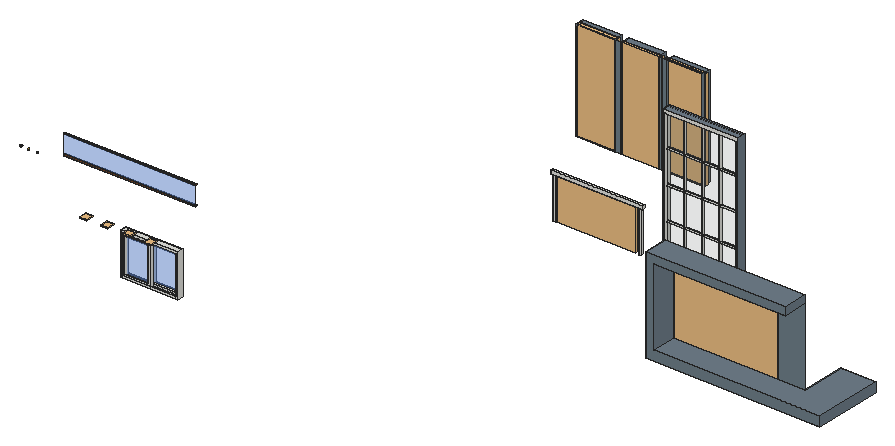
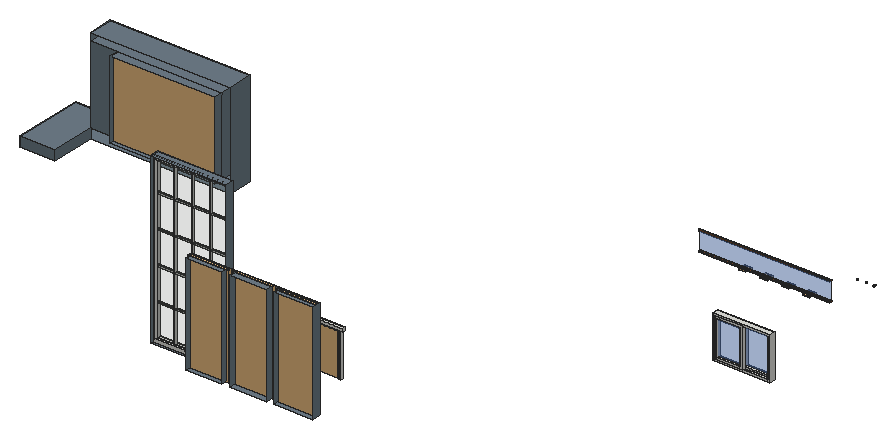
# SketchUp Ruby script. Lengths in inches.
U = 1.inch
M = Sketchup.active_model
def pt(a) = Geom::Point3d.new(a.map { |v| v * U })
def face(e, loops, mat)
  f = e.add_face(loops[0].map { |a| pt(a) })
  loops[1..].each { |l| e.add_face(l.map { |a| pt(a) }).erase! }
  f.material = f.back_material = mat if mat
  f
end
# faces: each face lists its corners as indices into pts; further lists are holes
def faces(e, pts, list, mat = nil) = list.each { |f| face(e, (f[0].is_a?(Array) ? f : [f]).map { |l| l.map { |i| pts[i] } }, mat) }
# xy, xz, yz: faces in a plane at the given z, y or x. An outline is a flat list of corners, or four numbers for a rectangle; further outlines are holes
def ring(l) = l.size == 4 ? [[l[0], l[1]], [l[2], l[1]], [l[2], l[3]], [l[0], l[3]]] : l.each_slice(2).to_a
def flat(e, list, mat, &to3) = list.each { |f| face(e, (f[0].is_a?(Array) ? f : [f]).map { |l| ring(l).map { |u, v| to3.(u, v) } }, mat) }
def xy(e, z, list, mat = nil) = flat(e, list, mat) { |x, y| [x, y, z] }
def xz(e, y, list, mat = nil) = flat(e, list, mat) { |x, z| [x, y, z] }
def yz(e, x, list, mat = nil) = flat(e, list, mat) { |y, z| [x, y, z] }
def lines(e, pts, list) = list.each { |a, b| e.add_line(pt(pts[a]), pt(pts[b])) }
# prism: a flat outline (further loops are holes) pulled along v
def prism(e, loops, v, mat = nil)
  f = face(e, loops, mat); d = Geom::Vector3d.new(v.map { |x| x * U })
  f.pushpull(f.normal.samedirection?(d) ? d.length : -d.length)
end
def box(e, o, s, mat = nil) = prism(e, [[o, [o[0] + s[0], o[1], o[2]], [o[0] + s[0], o[1] + s[1], o[2]], [o[0], o[1] + s[1], o[2]]]], [0, 0, s[2]], mat)
def at(x, y, z, deg = 0) = Geom::Transformation.translation(pt([x, y, z])) * Geom::Transformation.rotation(ORIGIN, Z_AXIS, deg.degrees)
def axes(o, x, y, z) = Geom::Transformation.new([*x, 0, *y, 0, *z, 0, *pt(o).to_a, 1])
def part(name) = M.definitions.add(name)
# library, detail: a bought-in or finely detailed component or shape, given as its bounding box
def library(name, o, s) = part(name).tap { |d| box(d.entities, o, s) }
def detail(e, o, s) = box(e.add_group.entities, o, s)
def put(e, d, t, mat = nil) = e.add_instance(d, t).tap { |i| i.material = mat if mat }
def group(e, t, mat = nil) = e.add_group.tap { |g| g.transformation = t; g.material = mat if mat }.entities
root = M.entities
M.materials.add("Heather_Cuffs").color = [111, 126, 137]
M.materials.add("[Color D04]").color = [255, 204, 50]
M.materials["[Color D04]"].alpha = 0.66
M.materials.add("[Color E05]").color = [255, 255, 0]
M.materials.add("[Translucent Glass Blue]").color = [100, 149, 237]
M.materials["[Translucent Glass Blue]"].alpha = 0.5
M.materials.add("[Translucent Glass Gray]1").color = [120, 128, 125]
M.materials["[Translucent Glass Gray]1"].alpha = 0.1875
M.materials.add("[Wood Veneer 01]").color = [120, 70, 37]
c1 = part("Group\#58")
box(c1.entities,[0,0,0],[0.79,51.97,0.79])
c2 = part("Group\#67")
box(c2.entities,[0,0,0],[0.79,0.79,79.53])
c3 = part("Group\#8")
xy(c3.entities,0,[[0,0,19.69,39.37]])
c4 = part("Group\#9")
prism(c4.entities,[[[45.28,43.31,0],[45.28,0,0],[21.65,0,0],[21.65,43.31,0]],[[23.62,41.34,0],[23.62,1.97,0],[43.31,1.97,0],[43.31,41.34,0]]],[0,0,1.97])
c5 = part("Group\#13")
g1 = group(c5.entities,at(1.97,1.97,0))
put(g1,c3,at(1.97,1.97,0.98),"[Translucent Glass Blue]")
put(g1,c4,at(-21.65,0,0))
g2 = group(c5.entities,at(23.62,1.97,1.97))
put(g2,c3,at(1.97,1.97,0.98),"[Translucent Glass Blue]")
put(g2,c4,at(-21.65,0,0))
g3 = group(c5.entities,at(0,0,3.9375))
prism(g3,[[[0,47.24,-3.9375],[49.21,47.24,-3.9375],[49.21,0,-3.9375],[0,0,-3.9375]],[[1.97,1.97,-3.9375],[47.24,1.97,-3.9375],[47.24,45.28,-3.9375],[1.97,45.28,-3.9375]]],[0,0,3.9375])
c6 = part("Group43\#1")
box(c6.entities,[916.08,245.78,188.26],[2.36,2.36,22.23])
c7 = part("Group44\#1")
box(c7.entities,[1010.04,245.78,188.26],[2.36,2.36,22.23])
c8 = library("Group47\#1",[920.98,246.17,188.26],[82.61,1.57,22.23])
c9 = library("okno",[0,0,0],[1.97,20.83,48.43])
c10 = library("normal+window",[0,0,0],[4.84,65.35,84.65])
c11 = part("Group46\#1")
box(c11.entities,[916.08,245.58,210.49],[96.32,2.75,1.77])
c12 = part("Group\#7")
box(c12.entities,[0,0,0],[132.53,1.81,1])
prism(root,[[[35.62,61.46,262.86],[35.61,61.72,262.86],[35.68,61.97,262.86],[35.8,62.2,262.86],[35.99,62.39,262.86],[36.21,62.52,262.86],[36.46,62.59,262.86],[36.72,62.6,262.86],[36.97,62.53,262.86],[37.2,62.41,262.86],[37.39,62.22,262.86],[37.52,62,262.86],[37.59,61.75,262.86],[37.6,61.49,262.86],[37.53,61.23,262.86],[37.41,61.01,262.86],[37.23,60.82,262.86],[37,60.68,262.86],[36.75,60.61,262.86],[36.49,60.61,262.86],[36.24,60.67,262.86],[36.01,60.8,262.86],[35.82,60.98,262.86],[35.6875,61.21,262.86]]],[0,0,1],"[Color D04]")
prism(root,[[[26.62,61.46,262.86],[26.61,61.72,262.86],[26.68,61.97,262.86],[26.8,62.2,262.86],[26.99,62.39,262.86],[27.21,62.52,262.86],[27.46,62.59,262.86],[27.72,62.6,262.86],[27.97,62.53,262.86],[28.2,62.41,262.86],[28.39,62.22,262.86],[28.52,62,262.86],[28.59,61.75,262.86],[28.6,61.49,262.86],[28.53,61.23,262.86],[28.41,61.01,262.86],[28.23,60.82,262.86],[28,60.68,262.86],[27.75,60.61,262.86],[27.49,60.61,262.86],[27.24,60.67,262.86],[27.01,60.8,262.86],[26.82,60.98,262.86],[26.6875,61.21,262.86]]],[0,0,1],"[Color D04]")
xy(root,158.93,[[447.88,333.96,522.88,342.96]],"Heather_Cuffs")
xy(root,209.8,[[290.7,420.96,329.6,429.96],[336.74,420.96,373.65,429.96],[381.73,420.96,417.7,429.96]],"Heather_Cuffs")
xy(root,225,[[569.63,194.96,675.0625,203.96]],"Heather_Cuffs")
xy(root,262.86,[[19.49,60.61,19.24,60.67,19.01,60.8,18.82,60.98,18.6875,61.21,18.62,61.46,18.61,61.72,18.68,61.97,18.8,62.2,18.99,62.39,19.21,62.52,19.46,62.59,19.72,62.6,19.97,62.53,20.2,62.41,20.39,62.22,20.52,62,20.59,61.75,20.6,61.49,20.53,61.23,20.41,61.01,20.23,60.82,20,60.68,19.75,60.61]],"[Color D04]")
xy(root,263.86,[[19.49,60.61,19.75,60.61,20,60.68,20.23,60.82,20.41,61.01,20.53,61.23,20.6,61.49,20.59,61.75,20.52,62,20.39,62.22,20.2,62.41,19.97,62.53,19.72,62.6,19.46,62.59,19.21,62.52,18.99,62.39,18.8,62.2,18.68,61.97,18.61,61.72,18.62,61.46,18.6875,61.21,18.82,60.98,19.01,60.8,19.24,60.67]])
xy(root,302,[[586.58,178.82,586.06,178.89,585.58,179.09,585.16,179.41,584.84,179.82,584.64,180.3,584.58,180.82,584.64,181.34,584.84,181.82,585.16,182.23,585.58,182.55,586.06,182.75,586.58,182.82,587.09,182.75,587.58,182.55,587.99,182.23,588.31,181.82,588.51,181.34,588.58,180.82,588.51,180.3,588.31,179.82,587.99,179.41,587.58,179.09,587.09,178.89],[619.58,178.82,619.06,178.89,618.58,179.09,618.16,179.41,617.84,179.82,617.64,180.3,617.58,180.82,617.64,181.34,617.84,181.82,618.16,182.23,618.58,182.55,619.06,182.75,619.58,182.82,620.09,182.75,620.58,182.55,620.99,182.23,621.31,181.82,621.51,181.34,621.58,180.82,621.51,180.3,621.31,179.82,620.99,179.41,620.58,179.09,620.09,178.89],[651.58,178.82,651.06,178.89,650.58,179.09,650.16,179.41,649.84,179.82,649.64,180.3,649.58,180.82,649.64,181.34,649.84,181.82,650.16,182.23,650.58,182.55,651.06,182.75,651.58,182.82,652.09,182.75,652.58,182.55,652.99,182.23,653.31,181.82,653.51,181.34,653.58,180.82,653.51,180.3,653.31,179.82,652.99,179.41,652.58,179.09,652.09,178.89],[688.58,178.82,688.06,178.89,687.58,179.09,687.16,179.41,686.84,179.82,686.64,180.3,686.58,180.82,686.64,181.34,686.84,181.82,687.16,182.23,687.58,182.55,688.06,182.75,688.58,182.82,689.09,182.75,689.58,182.55,689.99,182.23,690.31,181.82,690.51,181.34,690.58,180.82,690.51,180.3,690.31,179.82,689.99,179.41,689.58,179.09,689.09,178.89]],"[Color E05]")
xy(root,303,[[586.58,178.82,587.09,178.89,587.58,179.09,587.99,179.41,588.31,179.82,588.51,180.3,588.58,180.82,588.51,181.34,588.31,181.82,587.99,182.23,587.58,182.55,587.09,182.75,586.58,182.82,586.06,182.75,585.58,182.55,585.16,182.23,584.84,181.82,584.64,181.34,584.58,180.82,584.64,180.3,584.84,179.82,585.16,179.41,585.58,179.09,586.06,178.89],[619.58,178.82,620.09,178.89,620.58,179.09,620.99,179.41,621.31,179.82,621.51,180.3,621.58,180.82,621.51,181.34,621.31,181.82,620.99,182.23,620.58,182.55,620.09,182.75,619.58,182.82,619.06,182.75,618.58,182.55,618.16,182.23,617.84,181.82,617.64,181.34,617.58,180.82,617.64,180.3,617.84,179.82,618.16,179.41,618.58,179.09,619.06,178.89],[651.58,178.82,652.09,178.89,652.58,179.09,652.99,179.41,653.31,179.82,653.51,180.3,653.58,180.82,653.51,181.34,653.31,181.82,652.99,182.23,652.58,182.55,652.09,182.75,651.58,182.82,651.06,182.75,650.58,182.55,650.16,182.23,649.84,181.82,649.64,181.34,649.58,180.82,649.64,180.3,649.84,179.82,650.16,179.41,650.58,179.09,651.06,178.89],[688.58,178.82,689.09,178.89,689.58,179.09,689.99,179.41,690.31,179.82,690.51,180.3,690.58,180.82,690.51,181.34,690.31,181.82,689.99,182.23,689.58,182.55,689.09,182.75,688.58,182.82,688.06,182.75,687.58,182.55,687.16,182.23,686.84,181.82,686.64,181.34,686.58,180.82,686.64,180.3,686.84,179.82,687.16,179.41,687.58,179.09,688.06,178.89]])
xy(root,303,[[569.63,194.96,675.0625,203.96]],"Heather_Cuffs")
xy(root,310.8,[[290.7,420.96,329.6,429.96],[336.74,420.96,373.65,429.96],[381.73,420.96,417.7,429.96]],"Heather_Cuffs")
xy(root,327.93,[[447.88,333.96,522.88,342.96]],"Heather_Cuffs")
xz(root,60.61,[[19.49,262.86,19.75,263.86]],"[Color D04]")
xz(root,87,[[42.47,253,175,271]],"[Translucent Glass Blue]")
xz(root,420.96,[[329.6,209.8,336.74,310.8],[373.65,209.8,381.73,310.8]],"Heather_Cuffs")
yz(root,290.7,[[420.96,209.8,429.96,310.8]],"Heather_Cuffs")
yz(root,329.6,[[420.96,209.8,429.96,310.8]],"Heather_Cuffs")
yz(root,336.74,[[420.96,209.8,429.96,310.8]],"Heather_Cuffs")
yz(root,373.65,[[420.96,209.8,429.96,310.8]],"Heather_Cuffs")
yz(root,381.73,[[420.96,209.8,429.96,310.8]],"Heather_Cuffs")
yz(root,417.7,[[420.96,209.8,429.96,310.8]],"Heather_Cuffs")
yz(root,447.88,[[333.96,158.93,342.96,327.93]],"Heather_Cuffs")
yz(root,522.88,[[333.96,158.93,342.96,327.93]],"Heather_Cuffs")
yz(root,569.63,[[194.96,225,203.96,303]],"Heather_Cuffs")
yz(root,675.0625,[[194.96,225,203.96,303]],"Heather_Cuffs")
p = [[19.49,60.61,263.86],[19.24,60.67,263.86],[19.24,60.67,262.86],[19.49,60.61,262.86],[20,60.68,263.86],[19.75,60.61,263.86],
  [19.75,60.61,262.86],[20,60.68,262.86],[19.01,60.8,263.86],[19.01,60.8,262.86],[20.23,60.82,263.86],[20.23,60.82,262.86],
  [18.82,60.98,263.86],[18.82,60.98,262.86],[20.41,61.01,263.86],[20.41,61.01,262.86],[18.6875,61.21,263.86],[18.6875,61.21,262.86],
  [20.53,61.23,263.86],[20.53,61.23,262.86],[18.62,61.46,263.86],[18.62,61.46,262.86],[20.6,61.49,263.86],[20.6,61.49,262.86],
  [18.61,61.72,263.86],[18.61,61.72,262.86],[20.59,61.75,263.86],[20.59,61.75,262.86],[18.68,61.97,263.86],[18.68,61.97,262.86],
  [20.52,62,263.86],[20.52,62,262.86],[18.8,62.2,263.86],[18.8,62.2,262.86],[20.39,62.22,263.86],[20.39,62.22,262.86],
  [18.99,62.39,263.86],[18.99,62.39,262.86],[20.2,62.41,263.86],[20.2,62.41,262.86],[19.21,62.52,263.86],[19.21,62.52,262.86],
  [19.97,62.53,263.86],[19.97,62.53,262.86],[19.46,62.59,263.86],[19.46,62.59,262.86],[19.72,62.6,263.86],[19.72,62.6,262.86],
  [586.58,178.82,303],[586.06,178.89,303],[586.06,178.89,302],[586.58,178.82,302],[587.09,178.89,303],[587.09,178.89,302],
  [619.58,178.82,303],[619.06,178.89,303],[619.06,178.89,302],[619.58,178.82,302],[620.09,178.89,303],[620.09,178.89,302],
  [651.58,178.82,303],[651.06,178.89,303],[651.06,178.89,302],[651.58,178.82,302],[652.09,178.89,303],[652.09,178.89,302],
  [688.58,178.82,303],[688.06,178.89,303],[688.06,178.89,302],[688.58,178.82,302],[689.09,178.89,303],[689.09,178.89,302],
  [585.58,179.09,303],[585.58,179.09,302],[587.58,179.09,303],[587.58,179.09,302],[618.58,179.09,303],[618.58,179.09,302],
  [620.58,179.09,303],[620.58,179.09,302],[650.58,179.09,303],[650.58,179.09,302],[652.58,179.09,303],[652.58,179.09,302],
  [687.58,179.09,303],[687.58,179.09,302],[689.58,179.09,303],[689.58,179.09,302],[585.16,179.41,303],[585.16,179.41,302],
  [587.99,179.41,303],[587.99,179.41,302],[618.16,179.41,303],[618.16,179.41,302],[620.99,179.41,303],[620.99,179.41,302],
  [650.16,179.41,303],[650.16,179.41,302],[652.99,179.41,303],[652.99,179.41,302],[687.16,179.41,303],[687.16,179.41,302],
  [689.99,179.41,303],[689.99,179.41,302],[584.84,179.82,303],[584.84,179.82,302],[588.31,179.82,303],[588.31,179.82,302],
  [617.84,179.82,303],[617.84,179.82,302],[621.31,179.82,303],[621.31,179.82,302],[649.84,179.82,303],[649.84,179.82,302],
  [653.31,179.82,303],[653.31,179.82,302],[686.84,179.82,303],[686.84,179.82,302],[690.31,179.82,303],[690.31,179.82,302],
  [584.64,180.3,303],[584.64,180.3,302],[588.51,180.3,303],[588.51,180.3,302],[617.64,180.3,303],[617.64,180.3,302],
  [621.51,180.3,303],[621.51,180.3,302],[649.64,180.3,303],[649.64,180.3,302],[653.51,180.3,303],[653.51,180.3,302],
  [686.64,180.3,303],[686.64,180.3,302],[690.51,180.3,303],[690.51,180.3,302],[584.58,180.82,303],[584.58,180.82,302],
  [588.58,180.82,303],[588.58,180.82,302],[617.58,180.82,303],[617.58,180.82,302],[621.58,180.82,303],[621.58,180.82,302],
  [649.58,180.82,303],[649.58,180.82,302],[653.58,180.82,303],[653.58,180.82,302],[686.58,180.82,303],[686.58,180.82,302],
  [690.58,180.82,303],[690.58,180.82,302],[584.64,181.34,303],[584.64,181.34,302],[588.51,181.34,303],[588.51,181.34,302],
  [617.64,181.34,303],[617.64,181.34,302],[621.51,181.34,303],[621.51,181.34,302],[649.64,181.34,303],[649.64,181.34,302],
  [653.51,181.34,303],[653.51,181.34,302],[686.64,181.34,303],[686.64,181.34,302],[690.51,181.34,303],[690.51,181.34,302],
  [584.84,181.82,303],[584.84,181.82,302],[588.31,181.82,303],[588.31,181.82,302],[617.84,181.82,303],[617.84,181.82,302],
  [621.31,181.82,303],[621.31,181.82,302],[649.84,181.82,303],[649.84,181.82,302],[653.31,181.82,303],[653.31,181.82,302],
  [686.84,181.82,303],[686.84,181.82,302],[690.31,181.82,303],[690.31,181.82,302],[585.16,182.23,303],[585.16,182.23,302],
  [587.99,182.23,303],[587.99,182.23,302],[618.16,182.23,303],[618.16,182.23,302],[620.99,182.23,303],[620.99,182.23,302],
  [650.16,182.23,303],[650.16,182.23,302],[652.99,182.23,303],[652.99,182.23,302],[687.16,182.23,303],[687.16,182.23,302],
  [689.99,182.23,303],[689.99,182.23,302],[585.58,182.55,303],[585.58,182.55,302],[587.58,182.55,303],[587.58,182.55,302],
  [618.58,182.55,303],[618.58,182.55,302],[620.58,182.55,303],[620.58,182.55,302],[650.58,182.55,303],[650.58,182.55,302],
  [652.58,182.55,303],[652.58,182.55,302],[687.58,182.55,303],[687.58,182.55,302],[689.58,182.55,303],[689.58,182.55,302],
  [586.06,182.75,303],[586.06,182.75,302],[587.09,182.75,303],[587.09,182.75,302],[619.06,182.75,303],[619.06,182.75,302],
  [620.09,182.75,303],[620.09,182.75,302],[651.06,182.75,303],[651.06,182.75,302],[652.09,182.75,303],[652.09,182.75,302],
  [688.06,182.75,303],[688.06,182.75,302],[689.09,182.75,303],[689.09,182.75,302],[586.58,182.82,303],[586.58,182.82,302],
  [619.58,182.82,303],[619.58,182.82,302],[651.58,182.82,303],[651.58,182.82,302],[688.58,182.82,303],[688.58,182.82,302]]
faces(root,p,[[0,1,2,3],[4,5,6,7],[1,8,9,2],[10,4,7,11],[8,12,13,9],[14,10,11,15],[12,16,17,13],[18,14,15,19],
  [16,20,21,17],[22,18,19,23],[20,24,25,21],[26,22,23,27],[24,28,29,25],[30,26,27,31],[28,32,33,29],[34,30,31,35],
  [32,36,37,33],[38,34,35,39],[36,40,41,37],[42,38,39,43],[40,44,45,41],[46,42,43,47],[44,46,47,45]],"[Color D04]")
faces(root,p,[[48,49,50,51],[52,48,51,53],[54,55,56,57],[58,54,57,59],[60,61,62,63],[64,60,63,65],[66,67,68,69],[70,66,69,71],
  [49,72,73,50],[74,52,53,75],[55,76,77,56],[78,58,59,79],[61,80,81,62],[82,64,65,83],[67,84,85,68],[86,70,71,87],
  [72,88,89,73],[90,74,75,91],[76,92,93,77],[94,78,79,95],[80,96,97,81],[98,82,83,99],[84,100,101,85],[102,86,87,103],
  [88,104,105,89],[106,90,91,107],[92,108,109,93],[110,94,95,111],[96,112,113,97],[114,98,99,115],[100,116,117,101],[118,102,103,119],
  [104,120,121,105],[122,106,107,123],[108,124,125,109],[126,110,111,127],[112,128,129,113],[130,114,115,131],[116,132,133,117],[134,118,119,135],
  [120,136,137,121],[138,122,123,139],[124,140,141,125],[142,126,127,143],[128,144,145,129],[146,130,131,147],[132,148,149,133],[150,134,135,151],
  [136,152,153,137],[154,138,139,155],[140,156,157,141],[158,142,143,159],[144,160,161,145],[162,146,147,163],[148,164,165,149],[166,150,151,167],
  [152,168,169,153],[170,154,155,171],[156,172,173,157],[174,158,159,175],[160,176,177,161],[178,162,163,179],[164,180,181,165],[182,166,167,183],
  [168,184,185,169],[186,170,171,187],[172,188,189,173],[190,174,175,191],[176,192,193,177],[194,178,179,195],[180,196,197,181],[198,182,183,199],
  [184,200,201,185],[202,186,187,203],[188,204,205,189],[206,190,191,207],[192,208,209,193],[210,194,195,211],[196,212,213,197],[214,198,199,215],
  [200,216,217,201],[218,202,203,219],[204,220,221,205],[222,206,207,223],[208,224,225,209],[226,210,211,227],[212,228,229,213],[230,214,215,231],
  [216,232,233,217],[232,218,219,233],[220,234,235,221],[234,222,223,235],[224,236,237,225],[236,226,227,237],[228,238,239,229],[238,230,231,239]])
detail(root,[87.3,50.41,227.74],[7.44,7.43,1])
detail(root,[108.9,50.41,227.74],[7.43,7.43,1])
detail(root,[130.49,50.41,227.74],[7.44,7.43,1])
detail(root,[152.09,50.41,227.74],[7.43,7.43,1])
g4 = group(root,at(447.88,333.96,158.93))
g5 = group(g4,at(75,0,0))
g6 = group(g5,at(-2.14,3.46,3.22))
xz(g6,0,[[-70.71,0,0,162.5625]],"[Translucent Glass Gray]1")
g7 = group(g5,at(0,0,0))
xy(g7,0,[[-75,0,0,6.3]])
xy(g7,3.22,[[-72.86,0,-2.14,3.46],[-72.86,3.46,-2.14,6.3]])
xy(g7,165.78,[[-72.86,0,-2.14,3.46],[-72.86,3.46,-2.14,6.3]])
xy(g7,169,[[-75,0,0,6.3]])
xz(g7,0,[[[-75,0,0,169],[-72.86,3.22,-2.14,165.78]]])
xz(g7,6.3,[[[-75,0,0,169],[-72.86,3.22,-2.14,165.78]]])
yz(g7,-75,[[0,0,6.3,169]])
yz(g7,-72.86,[[0,3.22,3.46,165.78],[3.46,3.22,6.3,165.78]])
yz(g7,-2.14,[[0,3.22,3.46,165.78],[3.46,3.22,6.3,165.78]])
yz(g7,0,[[0,0,6.3,169]])
g8 = group(g4,at(72.86,1.89,3.22))
put(g8,c1,axes([0,0,30.84],[0,2,0],[-1.36071,0,0],[0,0,2.0441]))
put(g8,c1,axes([0,0,63.77],[0,2,0],[-1.36071,0,0],[0,0,2.0441]))
put(g8,c2,axes([-16.83,0,0],[0,2,0],[-1.36071,0,0],[0,0,2.0441]))
put(g8,c2,axes([-34.79,0,0],[0,2,0],[-1.36071,0,0],[0,0,2.0441]))
put(g8,c2,axes([-52.75,0,0],[0,2,0],[-1.36071,0,0],[0,0,2.0441]))
g9 = group(g8,at(0,0,129.63))
box(g9,[-70.71,0,0],[70.71,1.57,1.61])
put(g8,c1,axes([0,0,96.7],[0,2,0],[-1.36071,0,0],[0,0,2.0441]))
put(root,c5,axes([99.45,87,205],[1.17915,0,0],[0,0,-0.90737],[0,1.56718,0]))
put(root,c6,axes([-542.66,98.01,-173.35],[0.9604,0,0],[0,0.9604,0],[0,0,1.9208]))
put(root,c7,axes([-546.2,98.01,-173.35],[0.9604,0,0],[0,0.9604,0],[0,0,1.9208]))
put(root,c8,axes([-543.8,97.83,-173.35],[0.9604,0,0],[0,0.9604,0],[0,0,1.9208]))
put(root,c9,axes([376.55,420.96,209.8],[0,1.4718,0],[-1.96475,0,0],[0,0,2.08569]))
put(root,c9,axes([331.63,422.45,209.8],[0,1.4718,0],[-1.96475,0,0],[0,0,2.08569]))
put(root,c9,axes([419.74,422.45,209.8],[0,1.4718,0],[-1.96475,0,0],[0,0,2.08569]))
g10 = group(root,at(561.22,194.96,214.89),"Heather_Cuffs")
xy(g10,0,[[0,-25,0,0,141,0,141,45,176,45,176,-25]],"Heather_Cuffs")
xy(g10,10.11,[[8.41,-25,176,-25,176,45,141,45,141,0,8.41,0]],"Heather_Cuffs")
xy(g10,88.11,[[8.41,-25,141,0]],"Heather_Cuffs")
xy(g10,96,[[0,-25,141,0]],"Heather_Cuffs")
xz(g10,-25,[[0,0,176,0,176,10.11,8.41,10.11,8.41,88.11,141,88.11,141,96,0,96]],"Heather_Cuffs")
xz(g10,0,[[113.84,10.11,141,88.11]])
xz(g10,45,[[141,0,176,10.11]],"Heather_Cuffs")
yz(g10,0,[[-25,0,0,96]],"Heather_Cuffs")
yz(g10,8.41,[[-25,10.11,0,88.11]],"Heather_Cuffs")
yz(g10,141,[[0,0,45,10.11],[-25,88.11,0,96]],"Heather_Cuffs")
yz(g10,176,[[-25,0,45,10.11]],"Heather_Cuffs")
put(root,c10,axes([675.0625,194.96,225],[0,1.07568,0],[-1.61319,0,0],[0,0,0.90343]))
put(root,c11,axes([-543.8,96.875,-173.35],[0.9604,0,0],[0,0.9604,0],[0,0,1.9208]))
g11 = group(root,at(42.47,87,252))
put(g11,c12,at(0,0,0),"[Wood Veneer 01]")
put(g11,c12,at(0,0,19),"[Wood Veneer 01]")
